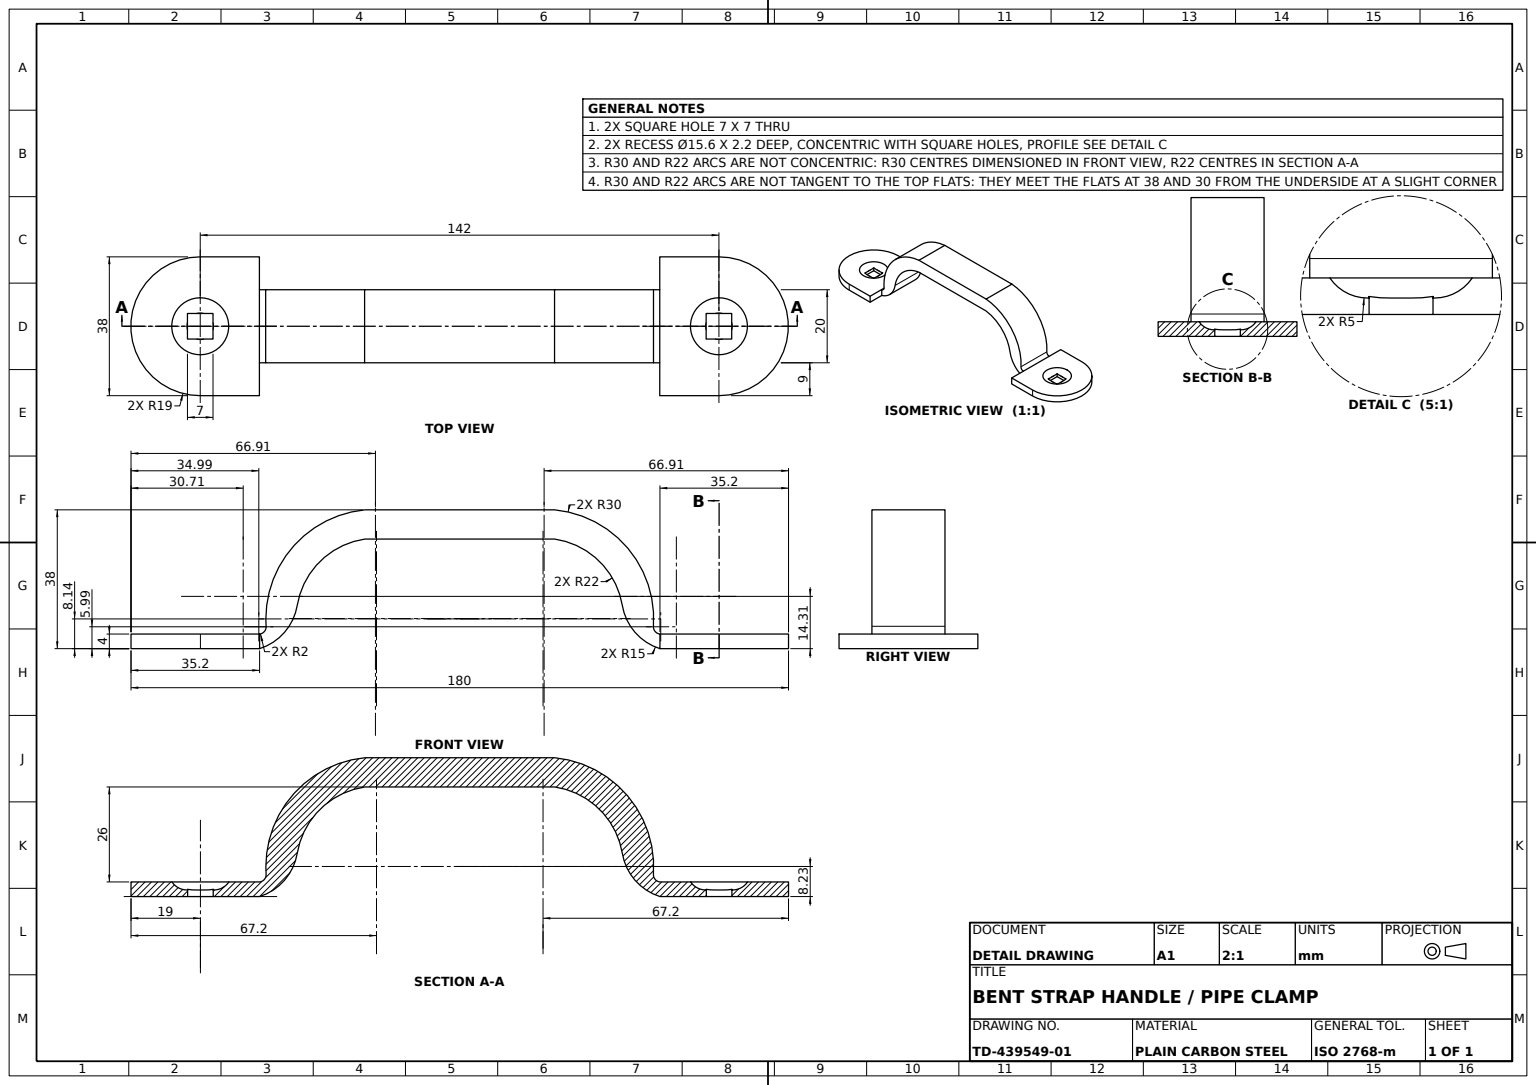
ISO-10303-21;
HEADER;
FILE_DESCRIPTION((''),'2;1');
FILE_NAME('','',(''),(''),'','','');
FILE_SCHEMA(('AUTOMOTIVE_DESIGN'));
ENDSEC;
DATA;
#1=APPLICATION_CONTEXT('');
#2=PRODUCT_CONTEXT('',#1,'mechanical');
#3=PRODUCT('','','',(#2));
#4=PRODUCT_DEFINITION_FORMATION('','',#3);
#5=PRODUCT_DEFINITION_CONTEXT('',#1,'design');
#6=PRODUCT_DEFINITION('','',#4,#5);
#7=PRODUCT_DEFINITION_SHAPE('','',#6);
#8=(LENGTH_UNIT()NAMED_UNIT(*)SI_UNIT(.MILLI.,.METRE.));
#9=(NAMED_UNIT(*)PLANE_ANGLE_UNIT()SI_UNIT($,.RADIAN.));
#10=(NAMED_UNIT(*)SI_UNIT($,.STERADIAN.)SOLID_ANGLE_UNIT());
#11=UNCERTAINTY_MEASURE_WITH_UNIT(LENGTH_MEASURE(1.E-05),#8,'distance_accuracy_value','');
#12=(GEOMETRIC_REPRESENTATION_CONTEXT(3)GLOBAL_UNCERTAINTY_ASSIGNED_CONTEXT((#11))GLOBAL_UNIT_ASSIGNED_CONTEXT((#8,#9,#10))REPRESENTATION_CONTEXT('',''));
#13=CARTESIAN_POINT('',(-16.2,4.,-19.));
#14=VERTEX_POINT('',#13);
#15=CARTESIAN_POINT('',(-16.2,4.,19.));
#16=VERTEX_POINT('',#15);
#17=CARTESIAN_POINT('',(-16.2,4.,0.));
#18=DIRECTION('',(0.,1.,0.));
#19=DIRECTION('',(0.,0.,1.));
#20=AXIS2_PLACEMENT_3D('',#17,#18,#19);
#21=CIRCLE('',#20,19.);
#22=EDGE_CURVE('',#14,#16,#21,.T.);
#23=ORIENTED_EDGE('',*,*,#22,.T.);
#24=CARTESIAN_POINT('',(0.,4.,19.));
#25=VERTEX_POINT('',#24);
#26=DIRECTION('',(1.,0.,0.));
#27=VECTOR('',#26,1000.);
#28=LINE('',#24,#27);
#29=EDGE_CURVE('',#16,#25,#28,.T.);
#30=ORIENTED_EDGE('',*,*,#29,.T.);
#31=CARTESIAN_POINT('',(0.,4.,10.));
#32=VERTEX_POINT('',#31);
#33=DIRECTION('',(0.,0.,-1.));
#34=VECTOR('',#33,1000.);
#35=LINE('',#24,#34);
#36=EDGE_CURVE('',#25,#32,#35,.T.);
#37=ORIENTED_EDGE('',*,*,#36,.T.);
#38=CARTESIAN_POINT('',(0.,4.,-10.));
#39=VERTEX_POINT('',#38);
#40=LINE('',#31,#34);
#41=EDGE_CURVE('',#32,#39,#40,.T.);
#42=ORIENTED_EDGE('',*,*,#41,.T.);
#43=CARTESIAN_POINT('',(0.,4.,-19.));
#44=VERTEX_POINT('',#43);
#45=EDGE_CURVE('',#39,#44,#35,.T.);
#46=ORIENTED_EDGE('',*,*,#45,.T.);
#47=DIRECTION('',(-1.,0.,0.));
#48=VECTOR('',#47,1000.);
#49=LINE('',#43,#48);
#50=EDGE_CURVE('',#44,#14,#49,.T.);
#51=ORIENTED_EDGE('',*,*,#50,.T.);
#52=EDGE_LOOP('',(#23,#30,#37,#42,#46,#51));
#53=FACE_OUTER_BOUND('',#52,.T.);
#54=CARTESIAN_POINT('',(-16.2,4.,7.8));
#55=VERTEX_POINT('',#54);
#56=CARTESIAN_POINT('',(-16.2,4.,-7.8));
#57=VERTEX_POINT('',#56);
#58=CIRCLE('',#20,7.8);
#59=EDGE_CURVE('',#55,#57,#58,.T.);
#60=ORIENTED_EDGE('',*,*,#59,.F.);
#61=EDGE_CURVE('',#57,#55,#58,.T.);
#62=ORIENTED_EDGE('',*,*,#61,.F.);
#63=EDGE_LOOP('',(#60,#62));
#64=FACE_BOUND('',#63,.T.);
#65=PLANE('',#20);
#66=ADVANCED_FACE('',(#53,#64),#65,.T.);
#67=CARTESIAN_POINT('',(107.814744,5.988438,-10.));
#68=VERTEX_POINT('',#67);
#69=CARTESIAN_POINT('',(107.819278,6.123019,-10.));
#70=VERTEX_POINT('',#69);
#71=CARTESIAN_POINT('',(109.814744,5.988438,-10.));
#72=AXIS2_PLACEMENT_3D('',#71,#33,#47);
#73=CIRCLE('',#72,2.);
#74=EDGE_CURVE('',#68,#70,#73,.T.);
#75=ORIENTED_EDGE('',*,*,#74,.T.);
#76=CARTESIAN_POINT('',(107.819278,6.123019,10.));
#77=VERTEX_POINT('',#76);
#78=LINE('',#76,#34);
#79=EDGE_CURVE('',#77,#70,#78,.T.);
#80=ORIENTED_EDGE('',*,*,#79,.F.);
#81=CARTESIAN_POINT('',(107.814744,5.988438,10.));
#82=VERTEX_POINT('',#81);
#83=CARTESIAN_POINT('',(109.814744,5.988438,10.));
#84=AXIS2_PLACEMENT_3D('',#83,#33,#47);
#85=CIRCLE('',#84,2.);
#86=EDGE_CURVE('',#82,#77,#85,.T.);
#87=ORIENTED_EDGE('',*,*,#86,.F.);
#88=LINE('',#81,#34);
#89=EDGE_CURVE('',#82,#68,#88,.T.);
#90=ORIENTED_EDGE('',*,*,#89,.T.);
#91=EDGE_LOOP('',(#75,#80,#87,#90));
#92=FACE_OUTER_BOUND('',#91,.T.);
#93=CYLINDRICAL_SURFACE('',#84,2.);
#94=ADVANCED_FACE('',(#92),#93,.F.);
#95=CARTESIAN_POINT('',(-12.7,1.8,1.061874));
#96=VERTEX_POINT('',#95);
#97=CARTESIAN_POINT('',(-12.7,1.8,-1.061874));
#98=VERTEX_POINT('',#97);
#99=CARTESIAN_POINT('',(-12.7,1.8,3.5));
#100=LINE('',#99,#34);
#101=EDGE_CURVE('',#96,#98,#100,.T.);
#102=ORIENTED_EDGE('',*,*,#101,.F.);
#103=CARTESIAN_POINT('',(-16.2,1.8,0.));
#104=AXIS2_PLACEMENT_3D('',#103,#18,#19);
#105=CIRCLE('',#104,3.657537);
#106=EDGE_CURVE('',#96,#98,#105,.T.);
#107=ORIENTED_EDGE('',*,*,#106,.T.);
#108=EDGE_LOOP('',(#102,#107));
#109=FACE_OUTER_BOUND('',#108,.T.);
#110=PLANE('',#104);
#111=ADVANCED_FACE('',(#109),#110,.T.);
#112=CARTESIAN_POINT('',(-19.7,0.,3.5));
#113=VERTEX_POINT('',#112);
#114=CARTESIAN_POINT('',(-12.7,0.,3.5));
#115=VERTEX_POINT('',#114);
#116=LINE('',#112,#27);
#117=EDGE_CURVE('',#113,#115,#116,.T.);
#118=ORIENTED_EDGE('',*,*,#117,.T.);
#119=CARTESIAN_POINT('',(-12.7,0.,-3.5));
#120=VERTEX_POINT('',#119);
#121=LINE('',#114,#34);
#122=EDGE_CURVE('',#115,#120,#121,.T.);
#123=ORIENTED_EDGE('',*,*,#122,.T.);
#124=CARTESIAN_POINT('',(-19.7,0.,-3.5));
#125=VERTEX_POINT('',#124);
#126=LINE('',#124,#48);
#127=EDGE_CURVE('',#120,#125,#126,.T.);
#128=ORIENTED_EDGE('',*,*,#127,.T.);
#129=VECTOR('',#19,1000.);
#130=LINE('',#112,#129);
#131=EDGE_CURVE('',#125,#113,#130,.T.);
#132=ORIENTED_EDGE('',*,*,#131,.T.);
#133=EDGE_LOOP('',(#118,#123,#128,#132));
#134=FACE_BOUND('',#133,.T.);
#135=CARTESIAN_POINT('',(0.,0.,-10.));
#136=VERTEX_POINT('',#135);
#137=CARTESIAN_POINT('',(0.,0.,-19.));
#138=VERTEX_POINT('',#137);
#139=CARTESIAN_POINT('',(0.,0.,19.));
#140=LINE('',#139,#34);
#141=EDGE_CURVE('',#136,#138,#140,.T.);
#142=ORIENTED_EDGE('',*,*,#141,.F.);
#143=CARTESIAN_POINT('',(0.,0.,10.));
#144=VERTEX_POINT('',#143);
#145=LINE('',#143,#34);
#146=EDGE_CURVE('',#144,#136,#145,.T.);
#147=ORIENTED_EDGE('',*,*,#146,.F.);
#148=VERTEX_POINT('',#139);
#149=EDGE_CURVE('',#148,#144,#140,.T.);
#150=ORIENTED_EDGE('',*,*,#149,.F.);
#151=CARTESIAN_POINT('',(-16.2,0.,19.));
#152=VERTEX_POINT('',#151);
#153=LINE('',#139,#27);
#154=EDGE_CURVE('',#152,#148,#153,.T.);
#155=ORIENTED_EDGE('',*,*,#154,.F.);
#156=CARTESIAN_POINT('',(-16.2,0.,-19.));
#157=VERTEX_POINT('',#156);
#158=CARTESIAN_POINT('',(-16.2,0.,0.));
#159=AXIS2_PLACEMENT_3D('',#158,#18,#19);
#160=CIRCLE('',#159,19.);
#161=EDGE_CURVE('',#157,#152,#160,.T.);
#162=ORIENTED_EDGE('',*,*,#161,.F.);
#163=LINE('',#137,#48);
#164=EDGE_CURVE('',#138,#157,#163,.T.);
#165=ORIENTED_EDGE('',*,*,#164,.F.);
#166=EDGE_LOOP('',(#142,#147,#150,#155,#162,#165));
#167=FACE_OUTER_BOUND('',#166,.T.);
#168=PLANE('',#159);
#169=ADVANCED_FACE('',(#134,#167),#168,.F.);
#170=CARTESIAN_POINT('',(109.6,0.,-19.));
#171=VERTEX_POINT('',#170);
#172=CARTESIAN_POINT('',(109.6,0.,-10.));
#173=VERTEX_POINT('',#172);
#174=CARTESIAN_POINT('',(109.6,0.,19.));
#175=LINE('',#174,#129);
#176=EDGE_CURVE('',#171,#173,#175,.T.);
#177=ORIENTED_EDGE('',*,*,#176,.T.);
#178=CARTESIAN_POINT('',(109.6,4.,-10.));
#179=VERTEX_POINT('',#178);
#180=VECTOR('',#18,1000.);
#181=LINE('',#172,#180);
#182=EDGE_CURVE('',#173,#179,#181,.T.);
#183=ORIENTED_EDGE('',*,*,#182,.T.);
#184=CARTESIAN_POINT('',(109.6,4.,-19.));
#185=VERTEX_POINT('',#184);
#186=CARTESIAN_POINT('',(109.6,4.,19.));
#187=LINE('',#186,#129);
#188=EDGE_CURVE('',#185,#179,#187,.T.);
#189=ORIENTED_EDGE('',*,*,#188,.F.);
#190=DIRECTION('',(0.,-1.,0.));
#191=VECTOR('',#190,1000.);
#192=LINE('',#184,#191);
#193=EDGE_CURVE('',#185,#171,#192,.T.);
#194=ORIENTED_EDGE('',*,*,#193,.T.);
#195=EDGE_LOOP('',(#177,#183,#189,#194));
#196=FACE_OUTER_BOUND('',#195,.T.);
#197=AXIS2_PLACEMENT_3D('',#186,#26,#33);
#198=PLANE('',#197);
#199=ADVANCED_FACE('',(#196),#198,.F.);
#200=CARTESIAN_POINT('',(122.3,1.8,-1.061874));
#201=VERTEX_POINT('',#200);
#202=CARTESIAN_POINT('',(122.3,1.8,1.061874));
#203=VERTEX_POINT('',#202);
#204=CARTESIAN_POINT('',(125.8,1.8,0.));
#205=AXIS2_PLACEMENT_3D('',#204,#18,#33);
#206=CIRCLE('',#205,3.657537);
#207=EDGE_CURVE('',#201,#203,#206,.T.);
#208=ORIENTED_EDGE('',*,*,#207,.T.);
#209=CARTESIAN_POINT('',(122.3,1.8,3.5));
#210=LINE('',#209,#129);
#211=EDGE_CURVE('',#201,#203,#210,.T.);
#212=ORIENTED_EDGE('',*,*,#211,.F.);
#213=EDGE_LOOP('',(#208,#212));
#214=FACE_OUTER_BOUND('',#213,.T.);
#215=AXIS2_PLACEMENT_3D('',#204,#190,#33);
#216=PLANE('',#215);
#217=ADVANCED_FACE('',(#214),#216,.F.);
#218=CARTESIAN_POINT('',(28.8,38.,10.));
#219=VERTEX_POINT('',#218);
#220=CARTESIAN_POINT('',(28.8,38.,-10.));
#221=VERTEX_POINT('',#220);
#222=LINE('',#218,#34);
#223=EDGE_CURVE('',#219,#221,#222,.T.);
#224=ORIENTED_EDGE('',*,*,#223,.T.);
#225=CARTESIAN_POINT('',(1.712725,8.141734,-10.));
#226=VERTEX_POINT('',#225);
#227=CARTESIAN_POINT('',(31.712725,8.141734,-10.));
#228=AXIS2_PLACEMENT_3D('',#227,#19,#47);
#229=CIRCLE('',#228,30.);
#230=EDGE_CURVE('',#221,#226,#229,.T.);
#231=ORIENTED_EDGE('',*,*,#230,.T.);
#232=CARTESIAN_POINT('',(1.712725,8.141734,10.));
#233=VERTEX_POINT('',#232);
#234=LINE('',#232,#34);
#235=EDGE_CURVE('',#233,#226,#234,.T.);
#236=ORIENTED_EDGE('',*,*,#235,.F.);
#237=CARTESIAN_POINT('',(31.712725,8.141734,10.));
#238=AXIS2_PLACEMENT_3D('',#237,#19,#47);
#239=CIRCLE('',#238,30.);
#240=EDGE_CURVE('',#219,#233,#239,.T.);
#241=ORIENTED_EDGE('',*,*,#240,.F.);
#242=EDGE_LOOP('',(#224,#231,#236,#241));
#243=FACE_OUTER_BOUND('',#242,.T.);
#244=AXIS2_PLACEMENT_3D('',#237,#33,#47);
#245=CYLINDRICAL_SURFACE('',#244,30.);
#246=ADVANCED_FACE('',(#243),#245,.T.);
#247=CARTESIAN_POINT('',(124.738126,1.8,3.5));
#248=VERTEX_POINT('',#247);
#249=CARTESIAN_POINT('',(125.8,1.8,3.657537));
#250=VERTEX_POINT('',#249);
#251=EDGE_CURVE('',#248,#250,#206,.T.);
#252=ORIENTED_EDGE('',*,*,#251,.T.);
#253=CARTESIAN_POINT('',(126.861874,1.8,3.5));
#254=VERTEX_POINT('',#253);
#255=EDGE_CURVE('',#250,#254,#206,.T.);
#256=ORIENTED_EDGE('',*,*,#255,.T.);
#257=LINE('',#209,#27);
#258=EDGE_CURVE('',#248,#254,#257,.T.);
#259=ORIENTED_EDGE('',*,*,#258,.F.);
#260=EDGE_LOOP('',(#252,#256,#259));
#261=FACE_OUTER_BOUND('',#260,.T.);
#262=ADVANCED_FACE('',(#261),#216,.F.);
#263=CARTESIAN_POINT('',(125.8,4.,7.8));
#264=VERTEX_POINT('',#263);
#265=CARTESIAN_POINT('',(125.8,6.8,3.657537));
#266=AXIS2_PLACEMENT_3D('',#265,#47,#19);
#267=CIRCLE('',#266,5.);
#268=EDGE_CURVE('',#250,#264,#267,.T.);
#269=ORIENTED_EDGE('',*,*,#268,.F.);
#270=ORIENTED_EDGE('',*,*,#251,.F.);
#271=CARTESIAN_POINT('',(122.3,1.969866,3.5));
#272=VERTEX_POINT('',#271);
#273=CARTESIAN_POINT('',(123.10603,1.817387,3.5));
#274=CARTESIAN_POINT('',(123.921472,1.8,3.5));
#275=B_SPLINE_CURVE_WITH_KNOTS('',3,(#271,#273,#274,#247),.UNSPECIFIED.,.F.,.F.,(4,4),(0.,0.002444036),.UNSPECIFIED.);
#276=EDGE_CURVE('',#272,#248,#275,.T.);
#277=ORIENTED_EDGE('',*,*,#276,.F.);
#278=CARTESIAN_POINT('',(122.3,1.8,1.878528));
#279=CARTESIAN_POINT('',(122.3,1.817387,2.69397));
#280=B_SPLINE_CURVE_WITH_KNOTS('',3,(#202,#278,#279,#271),.UNSPECIFIED.,.F.,.F.,(4,4),(0.,0.002444036),.UNSPECIFIED.);
#281=EDGE_CURVE('',#203,#272,#280,.T.);
#282=ORIENTED_EDGE('',*,*,#281,.F.);
#283=ORIENTED_EDGE('',*,*,#207,.F.);
#284=CARTESIAN_POINT('',(122.3,1.969866,-3.5));
#285=VERTEX_POINT('',#284);
#286=CARTESIAN_POINT('',(122.3,1.817387,-2.69397));
#287=CARTESIAN_POINT('',(122.3,1.8,-1.878528));
#288=B_SPLINE_CURVE_WITH_KNOTS('',3,(#284,#286,#287,#200),.UNSPECIFIED.,.F.,.F.,(4,4),(0.,0.002444036),.UNSPECIFIED.);
#289=EDGE_CURVE('',#285,#201,#288,.T.);
#290=ORIENTED_EDGE('',*,*,#289,.F.);
#291=CARTESIAN_POINT('',(124.738126,1.8,-3.5));
#292=VERTEX_POINT('',#291);
#293=CARTESIAN_POINT('',(123.921472,1.8,-3.5));
#294=CARTESIAN_POINT('',(123.10603,1.817387,-3.5));
#295=B_SPLINE_CURVE_WITH_KNOTS('',3,(#291,#293,#294,#284),.UNSPECIFIED.,.F.,.F.,(4,4),(0.,0.002444036),.UNSPECIFIED.);
#296=EDGE_CURVE('',#292,#285,#295,.T.);
#297=ORIENTED_EDGE('',*,*,#296,.F.);
#298=CARTESIAN_POINT('',(125.8,1.8,-3.657537));
#299=VERTEX_POINT('',#298);
#300=EDGE_CURVE('',#299,#292,#206,.T.);
#301=ORIENTED_EDGE('',*,*,#300,.F.);
#302=CARTESIAN_POINT('',(125.8,4.,-7.8));
#303=VERTEX_POINT('',#302);
#304=CARTESIAN_POINT('',(125.8,6.8,-3.657537));
#305=AXIS2_PLACEMENT_3D('',#304,#26,#33);
#306=CIRCLE('',#305,5.);
#307=EDGE_CURVE('',#299,#303,#306,.T.);
#308=ORIENTED_EDGE('',*,*,#307,.T.);
#309=CARTESIAN_POINT('',(125.8,4.,0.));
#310=AXIS2_PLACEMENT_3D('',#309,#18,#33);
#311=CIRCLE('',#310,7.8);
#312=EDGE_CURVE('',#303,#264,#311,.T.);
#313=ORIENTED_EDGE('',*,*,#312,.T.);
#314=EDGE_LOOP('',(#269,#270,#277,#282,#283,#290,#297,#301,#308,#313));
#315=FACE_OUTER_BOUND('',#314,.T.);
#316=CARTESIAN_POINT('',(125.8,6.8,0.));
#317=AXIS2_PLACEMENT_3D('',#316,#18,#19);
#318=TOROIDAL_SURFACE('',#317,3.657537,5.);
#319=ADVANCED_FACE('',(#315),#318,.F.);
#320=CARTESIAN_POINT('',(80.8,38.,10.));
#321=VERTEX_POINT('',#320);
#322=LINE('',#218,#48);
#323=EDGE_CURVE('',#321,#219,#322,.T.);
#324=ORIENTED_EDGE('',*,*,#323,.F.);
#325=CARTESIAN_POINT('',(80.8,38.,-10.));
#326=VERTEX_POINT('',#325);
#327=LINE('',#320,#34);
#328=EDGE_CURVE('',#321,#326,#327,.T.);
#329=ORIENTED_EDGE('',*,*,#328,.T.);
#330=LINE('',#220,#48);
#331=EDGE_CURVE('',#326,#221,#330,.T.);
#332=ORIENTED_EDGE('',*,*,#331,.T.);
#333=ORIENTED_EDGE('',*,*,#223,.F.);
#334=EDGE_LOOP('',(#324,#329,#332,#333));
#335=FACE_OUTER_BOUND('',#334,.T.);
#336=AXIS2_PLACEMENT_3D('',#218,#190,#26);
#337=PLANE('',#336);
#338=ADVANCED_FACE('',(#335),#337,.F.);
#339=EDGE_CURVE('',#264,#303,#311,.T.);
#340=ORIENTED_EDGE('',*,*,#339,.F.);
#341=ORIENTED_EDGE('',*,*,#312,.F.);
#342=EDGE_LOOP('',(#340,#341));
#343=FACE_BOUND('',#342,.T.);
#344=ORIENTED_EDGE('',*,*,#188,.T.);
#345=CARTESIAN_POINT('',(109.6,4.,10.));
#346=VERTEX_POINT('',#345);
#347=LINE('',#345,#34);
#348=EDGE_CURVE('',#346,#179,#347,.T.);
#349=ORIENTED_EDGE('',*,*,#348,.F.);
#350=VERTEX_POINT('',#186);
#351=EDGE_CURVE('',#346,#350,#187,.T.);
#352=ORIENTED_EDGE('',*,*,#351,.T.);
#353=CARTESIAN_POINT('',(125.8,4.,19.));
#354=VERTEX_POINT('',#353);
#355=LINE('',#186,#27);
#356=EDGE_CURVE('',#350,#354,#355,.T.);
#357=ORIENTED_EDGE('',*,*,#356,.T.);
#358=CARTESIAN_POINT('',(125.8,4.,-19.));
#359=VERTEX_POINT('',#358);
#360=CIRCLE('',#310,19.);
#361=EDGE_CURVE('',#354,#359,#360,.T.);
#362=ORIENTED_EDGE('',*,*,#361,.T.);
#363=LINE('',#184,#48);
#364=EDGE_CURVE('',#359,#185,#363,.T.);
#365=ORIENTED_EDGE('',*,*,#364,.T.);
#366=EDGE_LOOP('',(#344,#349,#352,#357,#362,#365));
#367=FACE_OUTER_BOUND('',#366,.T.);
#368=AXIS2_PLACEMENT_3D('',#309,#190,#33);
#369=PLANE('',#368);
#370=ADVANCED_FACE('',(#343,#367),#369,.F.);
#371=ORIENTED_EDGE('',*,*,#106,.F.);
#372=CARTESIAN_POINT('',(-12.7,1.969866,3.5));
#373=VERTEX_POINT('',#372);
#374=CARTESIAN_POINT('',(-12.7,1.817387,2.69397));
#375=CARTESIAN_POINT('',(-12.7,1.8,1.878528));
#376=B_SPLINE_CURVE_WITH_KNOTS('',3,(#372,#374,#375,#95),.UNSPECIFIED.,.F.,.F.,(4,4),(0.,0.002444036),.UNSPECIFIED.);
#377=EDGE_CURVE('',#373,#96,#376,.T.);
#378=ORIENTED_EDGE('',*,*,#377,.F.);
#379=CARTESIAN_POINT('',(-15.138126,1.8,3.5));
#380=VERTEX_POINT('',#379);
#381=CARTESIAN_POINT('',(-14.321472,1.8,3.5));
#382=CARTESIAN_POINT('',(-13.50603,1.817387,3.5));
#383=B_SPLINE_CURVE_WITH_KNOTS('',3,(#379,#381,#382,#372),.UNSPECIFIED.,.F.,.F.,(4,4),(0.,0.002444036),.UNSPECIFIED.);
#384=EDGE_CURVE('',#380,#373,#383,.T.);
#385=ORIENTED_EDGE('',*,*,#384,.F.);
#386=CARTESIAN_POINT('',(-16.2,1.8,3.657537));
#387=VERTEX_POINT('',#386);
#388=EDGE_CURVE('',#387,#380,#105,.T.);
#389=ORIENTED_EDGE('',*,*,#388,.F.);
#390=CARTESIAN_POINT('',(-16.2,6.8,3.657537));
#391=AXIS2_PLACEMENT_3D('',#390,#26,#33);
#392=CIRCLE('',#391,5.);
#393=EDGE_CURVE('',#55,#387,#392,.T.);
#394=ORIENTED_EDGE('',*,*,#393,.F.);
#395=ORIENTED_EDGE('',*,*,#59,.T.);
#396=CARTESIAN_POINT('',(-16.2,1.8,-3.657537));
#397=VERTEX_POINT('',#396);
#398=CARTESIAN_POINT('',(-16.2,6.8,-3.657537));
#399=AXIS2_PLACEMENT_3D('',#398,#47,#19);
#400=CIRCLE('',#399,5.);
#401=EDGE_CURVE('',#57,#397,#400,.T.);
#402=ORIENTED_EDGE('',*,*,#401,.T.);
#403=CARTESIAN_POINT('',(-15.138126,1.8,-3.5));
#404=VERTEX_POINT('',#403);
#405=EDGE_CURVE('',#404,#397,#105,.T.);
#406=ORIENTED_EDGE('',*,*,#405,.F.);
#407=CARTESIAN_POINT('',(-12.7,1.969866,-3.5));
#408=VERTEX_POINT('',#407);
#409=CARTESIAN_POINT('',(-13.50603,1.817387,-3.5));
#410=CARTESIAN_POINT('',(-14.321472,1.8,-3.5));
#411=B_SPLINE_CURVE_WITH_KNOTS('',3,(#407,#409,#410,#403),.UNSPECIFIED.,.F.,.F.,(4,4),(0.,0.002444036),.UNSPECIFIED.);
#412=EDGE_CURVE('',#408,#404,#411,.T.);
#413=ORIENTED_EDGE('',*,*,#412,.F.);
#414=CARTESIAN_POINT('',(-12.7,1.8,-1.878528));
#415=CARTESIAN_POINT('',(-12.7,1.817387,-2.69397));
#416=B_SPLINE_CURVE_WITH_KNOTS('',3,(#97,#414,#415,#407),.UNSPECIFIED.,.F.,.F.,(4,4),(0.,0.002444036),.UNSPECIFIED.);
#417=EDGE_CURVE('',#98,#408,#416,.T.);
#418=ORIENTED_EDGE('',*,*,#417,.F.);
#419=EDGE_LOOP('',(#371,#378,#385,#389,#394,#395,#402,#406,#413,#418));
#420=FACE_OUTER_BOUND('',#419,.T.);
#421=CARTESIAN_POINT('',(-16.2,6.8,0.));
#422=AXIS2_PLACEMENT_3D('',#421,#190,#33);
#423=TOROIDAL_SURFACE('',#422,3.657537,5.);
#424=ADVANCED_FACE('',(#420),#423,.F.);
#425=ORIENTED_EDGE('',*,*,#348,.T.);
#426=EDGE_CURVE('',#179,#68,#73,.T.);
#427=ORIENTED_EDGE('',*,*,#426,.T.);
#428=ORIENTED_EDGE('',*,*,#89,.F.);
#429=EDGE_CURVE('',#346,#82,#85,.T.);
#430=ORIENTED_EDGE('',*,*,#429,.F.);
#431=EDGE_LOOP('',(#425,#427,#428,#430));
#432=FACE_OUTER_BOUND('',#431,.T.);
#433=ADVANCED_FACE('',(#432),#93,.F.);
#434=CARTESIAN_POINT('',(99.296405,11.847852,-10.));
#435=VERTEX_POINT('',#434);
#436=CARTESIAN_POINT('',(114.092724,14.311374,-10.));
#437=AXIS2_PLACEMENT_3D('',#436,#19,#47);
#438=CIRCLE('',#437,15.);
#439=EDGE_CURVE('',#435,#173,#438,.T.);
#440=ORIENTED_EDGE('',*,*,#439,.T.);
#441=CARTESIAN_POINT('',(109.6,0.,10.));
#442=VERTEX_POINT('',#441);
#443=LINE('',#441,#34);
#444=EDGE_CURVE('',#442,#173,#443,.T.);
#445=ORIENTED_EDGE('',*,*,#444,.F.);
#446=CARTESIAN_POINT('',(99.296405,11.847852,10.));
#447=VERTEX_POINT('',#446);
#448=CARTESIAN_POINT('',(114.092724,14.311374,10.));
#449=AXIS2_PLACEMENT_3D('',#448,#19,#47);
#450=CIRCLE('',#449,15.);
#451=EDGE_CURVE('',#447,#442,#450,.T.);
#452=ORIENTED_EDGE('',*,*,#451,.F.);
#453=LINE('',#446,#34);
#454=EDGE_CURVE('',#447,#435,#453,.T.);
#455=ORIENTED_EDGE('',*,*,#454,.T.);
#456=EDGE_LOOP('',(#440,#445,#452,#455));
#457=FACE_OUTER_BOUND('',#456,.T.);
#458=AXIS2_PLACEMENT_3D('',#448,#33,#47);
#459=CYLINDRICAL_SURFACE('',#458,15.);
#460=ADVANCED_FACE('',(#457),#459,.T.);
#461=CARTESIAN_POINT('',(80.8,30.,10.));
#462=VERTEX_POINT('',#461);
#463=CARTESIAN_POINT('',(77.595137,8.234687,10.));
#464=AXIS2_PLACEMENT_3D('',#463,#33,#26);
#465=CIRCLE('',#464,22.);
#466=EDGE_CURVE('',#462,#447,#465,.T.);
#467=ORIENTED_EDGE('',*,*,#466,.F.);
#468=CARTESIAN_POINT('',(80.8,30.,-10.));
#469=VERTEX_POINT('',#468);
#470=LINE('',#461,#34);
#471=EDGE_CURVE('',#462,#469,#470,.T.);
#472=ORIENTED_EDGE('',*,*,#471,.T.);
#473=CARTESIAN_POINT('',(77.595137,8.234687,-10.));
#474=AXIS2_PLACEMENT_3D('',#473,#33,#26);
#475=CIRCLE('',#474,22.);
#476=EDGE_CURVE('',#469,#435,#475,.T.);
#477=ORIENTED_EDGE('',*,*,#476,.T.);
#478=ORIENTED_EDGE('',*,*,#454,.F.);
#479=EDGE_LOOP('',(#467,#472,#477,#478));
#480=FACE_OUTER_BOUND('',#479,.T.);
#481=AXIS2_PLACEMENT_3D('',#463,#33,#47);
#482=CYLINDRICAL_SURFACE('',#481,22.);
#483=ADVANCED_FACE('',(#480),#482,.F.);
#484=ORIENTED_EDGE('',*,*,#193,.F.);
#485=ORIENTED_EDGE('',*,*,#364,.F.);
#486=CARTESIAN_POINT('',(125.8,0.,-19.));
#487=VERTEX_POINT('',#486);
#488=LINE('',#358,#191);
#489=EDGE_CURVE('',#359,#487,#488,.T.);
#490=ORIENTED_EDGE('',*,*,#489,.T.);
#491=LINE('',#170,#48);
#492=EDGE_CURVE('',#487,#171,#491,.T.);
#493=ORIENTED_EDGE('',*,*,#492,.T.);
#494=EDGE_LOOP('',(#484,#485,#490,#493));
#495=FACE_OUTER_BOUND('',#494,.T.);
#496=AXIS2_PLACEMENT_3D('',#184,#19,#26);
#497=PLANE('',#496);
#498=ADVANCED_FACE('',(#495),#497,.F.);
#499=CARTESIAN_POINT('',(-19.7,1.8,-1.061874));
#500=VERTEX_POINT('',#499);
#501=CARTESIAN_POINT('',(-19.7,1.8,1.061874));
#502=VERTEX_POINT('',#501);
#503=CARTESIAN_POINT('',(-19.7,1.8,3.5));
#504=LINE('',#503,#129);
#505=EDGE_CURVE('',#500,#502,#504,.T.);
#506=ORIENTED_EDGE('',*,*,#505,.F.);
#507=EDGE_CURVE('',#500,#502,#105,.T.);
#508=ORIENTED_EDGE('',*,*,#507,.T.);
#509=EDGE_LOOP('',(#506,#508));
#510=FACE_OUTER_BOUND('',#509,.T.);
#511=ADVANCED_FACE('',(#510),#110,.T.);
#512=CARTESIAN_POINT('',(10.303595,11.847852,10.));
#513=VERTEX_POINT('',#512);
#514=CARTESIAN_POINT('',(-4.492724,14.311374,10.));
#515=AXIS2_PLACEMENT_3D('',#514,#19,#26);
#516=CIRCLE('',#515,15.);
#517=EDGE_CURVE('',#144,#513,#516,.T.);
#518=ORIENTED_EDGE('',*,*,#517,.F.);
#519=ORIENTED_EDGE('',*,*,#146,.T.);
#520=CARTESIAN_POINT('',(10.303595,11.847852,-10.));
#521=VERTEX_POINT('',#520);
#522=CARTESIAN_POINT('',(-4.492724,14.311374,-10.));
#523=AXIS2_PLACEMENT_3D('',#522,#19,#26);
#524=CIRCLE('',#523,15.);
#525=EDGE_CURVE('',#136,#521,#524,.T.);
#526=ORIENTED_EDGE('',*,*,#525,.T.);
#527=LINE('',#512,#34);
#528=EDGE_CURVE('',#513,#521,#527,.T.);
#529=ORIENTED_EDGE('',*,*,#528,.F.);
#530=EDGE_LOOP('',(#518,#519,#526,#529));
#531=FACE_OUTER_BOUND('',#530,.T.);
#532=AXIS2_PLACEMENT_3D('',#514,#33,#47);
#533=CYLINDRICAL_SURFACE('',#532,15.);
#534=ADVANCED_FACE('',(#531),#533,.T.);
#535=ORIENTED_EDGE('',*,*,#356,.F.);
#536=VERTEX_POINT('',#174);
#537=LINE('',#186,#191);
#538=EDGE_CURVE('',#350,#536,#537,.T.);
#539=ORIENTED_EDGE('',*,*,#538,.T.);
#540=CARTESIAN_POINT('',(125.8,0.,19.));
#541=VERTEX_POINT('',#540);
#542=LINE('',#174,#27);
#543=EDGE_CURVE('',#536,#541,#542,.T.);
#544=ORIENTED_EDGE('',*,*,#543,.T.);
#545=LINE('',#353,#191);
#546=EDGE_CURVE('',#354,#541,#545,.T.);
#547=ORIENTED_EDGE('',*,*,#546,.F.);
#548=EDGE_LOOP('',(#535,#539,#544,#547));
#549=FACE_OUTER_BOUND('',#548,.T.);
#550=AXIS2_PLACEMENT_3D('',#186,#33,#47);
#551=PLANE('',#550);
#552=ADVANCED_FACE('',(#549),#551,.F.);
#553=CARTESIAN_POINT('',(1.780722,6.123019,10.));
#554=VERTEX_POINT('',#553);
#555=EDGE_CURVE('',#233,#554,#239,.T.);
#556=ORIENTED_EDGE('',*,*,#555,.F.);
#557=ORIENTED_EDGE('',*,*,#235,.T.);
#558=CARTESIAN_POINT('',(1.780722,6.123019,-10.));
#559=VERTEX_POINT('',#558);
#560=EDGE_CURVE('',#226,#559,#229,.T.);
#561=ORIENTED_EDGE('',*,*,#560,.T.);
#562=LINE('',#553,#34);
#563=EDGE_CURVE('',#554,#559,#562,.T.);
#564=ORIENTED_EDGE('',*,*,#563,.F.);
#565=EDGE_LOOP('',(#556,#557,#561,#564));
#566=FACE_OUTER_BOUND('',#565,.T.);
#567=ADVANCED_FACE('',(#566),#245,.T.);
#568=LINE('',#31,#191);
#569=EDGE_CURVE('',#32,#144,#568,.T.);
#570=ORIENTED_EDGE('',*,*,#569,.T.);
#571=ORIENTED_EDGE('',*,*,#517,.T.);
#572=CARTESIAN_POINT('',(28.8,30.,10.));
#573=VERTEX_POINT('',#572);
#574=CARTESIAN_POINT('',(32.004863,8.234687,10.));
#575=AXIS2_PLACEMENT_3D('',#574,#33,#47);
#576=CIRCLE('',#575,22.);
#577=EDGE_CURVE('',#513,#573,#576,.T.);
#578=ORIENTED_EDGE('',*,*,#577,.T.);
#579=LINE('',#572,#27);
#580=EDGE_CURVE('',#573,#462,#579,.T.);
#581=ORIENTED_EDGE('',*,*,#580,.T.);
#582=ORIENTED_EDGE('',*,*,#466,.T.);
#583=ORIENTED_EDGE('',*,*,#451,.T.);
#584=LINE('',#441,#180);
#585=EDGE_CURVE('',#442,#346,#584,.T.);
#586=ORIENTED_EDGE('',*,*,#585,.T.);
#587=ORIENTED_EDGE('',*,*,#429,.T.);
#588=ORIENTED_EDGE('',*,*,#86,.T.);
#589=CARTESIAN_POINT('',(77.887275,8.141734,10.));
#590=AXIS2_PLACEMENT_3D('',#589,#19,#26);
#591=CIRCLE('',#590,30.);
#592=EDGE_CURVE('',#77,#321,#591,.T.);
#593=ORIENTED_EDGE('',*,*,#592,.T.);
#594=ORIENTED_EDGE('',*,*,#323,.T.);
#595=ORIENTED_EDGE('',*,*,#240,.T.);
#596=ORIENTED_EDGE('',*,*,#555,.T.);
#597=CARTESIAN_POINT('',(-0.214744,5.988438,10.));
#598=AXIS2_PLACEMENT_3D('',#597,#33,#26);
#599=CIRCLE('',#598,2.);
#600=EDGE_CURVE('',#554,#32,#599,.T.);
#601=ORIENTED_EDGE('',*,*,#600,.T.);
#602=EDGE_LOOP('',(#570,#571,#578,#581,#582,#583,#586,#587,#588,#593,#594,#595,#596,#601));
#603=FACE_OUTER_BOUND('',#602,.T.);
#604=PLANE('',#515);
#605=ADVANCED_FACE('',(#603),#604,.T.);
#606=CARTESIAN_POINT('',(-0.214744,5.988438,-10.));
#607=AXIS2_PLACEMENT_3D('',#606,#33,#26);
#608=CIRCLE('',#607,2.);
#609=EDGE_CURVE('',#559,#39,#608,.T.);
#610=ORIENTED_EDGE('',*,*,#609,.T.);
#611=ORIENTED_EDGE('',*,*,#41,.F.);
#612=ORIENTED_EDGE('',*,*,#600,.F.);
#613=ORIENTED_EDGE('',*,*,#563,.T.);
#614=EDGE_LOOP('',(#610,#611,#612,#613));
#615=FACE_OUTER_BOUND('',#614,.T.);
#616=AXIS2_PLACEMENT_3D('',#597,#33,#47);
#617=CYLINDRICAL_SURFACE('',#616,2.);
#618=ADVANCED_FACE('',(#615),#617,.F.);
#619=CARTESIAN_POINT('',(129.3,0.,-3.5));
#620=VERTEX_POINT('',#619);
#621=CARTESIAN_POINT('',(129.3,1.969866,-3.5));
#622=VERTEX_POINT('',#621);
#623=LINE('',#619,#180);
#624=EDGE_CURVE('',#620,#622,#623,.T.);
#625=ORIENTED_EDGE('',*,*,#624,.F.);
#626=CARTESIAN_POINT('',(129.3,0.,3.5));
#627=VERTEX_POINT('',#626);
#628=LINE('',#626,#34);
#629=EDGE_CURVE('',#627,#620,#628,.T.);
#630=ORIENTED_EDGE('',*,*,#629,.F.);
#631=CARTESIAN_POINT('',(129.3,1.969866,3.5));
#632=VERTEX_POINT('',#631);
#633=LINE('',#626,#180);
#634=EDGE_CURVE('',#627,#632,#633,.T.);
#635=ORIENTED_EDGE('',*,*,#634,.T.);
#636=CARTESIAN_POINT('',(129.3,1.8,1.061874));
#637=VERTEX_POINT('',#636);
#638=CARTESIAN_POINT('',(129.3,1.817387,2.69397));
#639=CARTESIAN_POINT('',(129.3,1.8,1.878528));
#640=B_SPLINE_CURVE_WITH_KNOTS('',3,(#631,#638,#639,#636),.UNSPECIFIED.,.F.,.F.,(4,4),(0.,0.002444036),.UNSPECIFIED.);
#641=EDGE_CURVE('',#632,#637,#640,.T.);
#642=ORIENTED_EDGE('',*,*,#641,.T.);
#643=CARTESIAN_POINT('',(129.3,1.8,-1.061874));
#644=VERTEX_POINT('',#643);
#645=CARTESIAN_POINT('',(129.3,1.8,3.5));
#646=LINE('',#645,#34);
#647=EDGE_CURVE('',#637,#644,#646,.T.);
#648=ORIENTED_EDGE('',*,*,#647,.T.);
#649=CARTESIAN_POINT('',(129.3,1.8,-1.878528));
#650=CARTESIAN_POINT('',(129.3,1.817387,-2.69397));
#651=B_SPLINE_CURVE_WITH_KNOTS('',3,(#643,#649,#650,#621),.UNSPECIFIED.,.F.,.F.,(4,4),(0.,0.002444036),.UNSPECIFIED.);
#652=EDGE_CURVE('',#644,#622,#651,.T.);
#653=ORIENTED_EDGE('',*,*,#652,.T.);
#654=EDGE_LOOP('',(#625,#630,#635,#642,#648,#653));
#655=FACE_OUTER_BOUND('',#654,.T.);
#656=AXIS2_PLACEMENT_3D('',#626,#26,#33);
#657=PLANE('',#656);
#658=ADVANCED_FACE('',(#655),#657,.F.);
#659=LINE('',#114,#180);
#660=EDGE_CURVE('',#115,#373,#659,.T.);
#661=ORIENTED_EDGE('',*,*,#660,.F.);
#662=ORIENTED_EDGE('',*,*,#117,.F.);
#663=CARTESIAN_POINT('',(-19.7,1.969866,3.5));
#664=VERTEX_POINT('',#663);
#665=LINE('',#112,#180);
#666=EDGE_CURVE('',#113,#664,#665,.T.);
#667=ORIENTED_EDGE('',*,*,#666,.T.);
#668=CARTESIAN_POINT('',(-17.261874,1.8,3.5));
#669=VERTEX_POINT('',#668);
#670=CARTESIAN_POINT('',(-18.89397,1.817387,3.5));
#671=CARTESIAN_POINT('',(-18.078528,1.8,3.5));
#672=B_SPLINE_CURVE_WITH_KNOTS('',3,(#663,#670,#671,#668),.UNSPECIFIED.,.F.,.F.,(4,4),(0.,0.002444036),.UNSPECIFIED.);
#673=EDGE_CURVE('',#664,#669,#672,.T.);
#674=ORIENTED_EDGE('',*,*,#673,.T.);
#675=LINE('',#503,#27);
#676=EDGE_CURVE('',#669,#380,#675,.T.);
#677=ORIENTED_EDGE('',*,*,#676,.T.);
#678=ORIENTED_EDGE('',*,*,#384,.T.);
#679=EDGE_LOOP('',(#661,#662,#667,#674,#677,#678));
#680=FACE_OUTER_BOUND('',#679,.T.);
#681=AXIS2_PLACEMENT_3D('',#112,#19,#26);
#682=PLANE('',#681);
#683=ADVANCED_FACE('',(#680),#682,.F.);
#684=ORIENTED_EDGE('',*,*,#676,.F.);
#685=EDGE_CURVE('',#669,#387,#105,.T.);
#686=ORIENTED_EDGE('',*,*,#685,.T.);
#687=ORIENTED_EDGE('',*,*,#388,.T.);
#688=EDGE_LOOP('',(#684,#686,#687));
#689=FACE_OUTER_BOUND('',#688,.T.);
#690=ADVANCED_FACE('',(#689),#110,.T.);
#691=CARTESIAN_POINT('',(126.861874,1.8,-3.5));
#692=VERTEX_POINT('',#691);
#693=CARTESIAN_POINT('',(128.49397,1.817387,-3.5));
#694=CARTESIAN_POINT('',(127.678528,1.8,-3.5));
#695=B_SPLINE_CURVE_WITH_KNOTS('',3,(#621,#693,#694,#691),.UNSPECIFIED.,.F.,.F.,(4,4),(0.,0.002444036),.UNSPECIFIED.);
#696=EDGE_CURVE('',#622,#692,#695,.T.);
#697=ORIENTED_EDGE('',*,*,#696,.F.);
#698=ORIENTED_EDGE('',*,*,#652,.F.);
#699=EDGE_CURVE('',#637,#644,#206,.T.);
#700=ORIENTED_EDGE('',*,*,#699,.F.);
#701=ORIENTED_EDGE('',*,*,#641,.F.);
#702=CARTESIAN_POINT('',(127.678528,1.8,3.5));
#703=CARTESIAN_POINT('',(128.49397,1.817387,3.5));
#704=B_SPLINE_CURVE_WITH_KNOTS('',3,(#253,#702,#703,#631),.UNSPECIFIED.,.F.,.F.,(4,4),(0.,0.002444036),.UNSPECIFIED.);
#705=EDGE_CURVE('',#254,#632,#704,.T.);
#706=ORIENTED_EDGE('',*,*,#705,.F.);
#707=ORIENTED_EDGE('',*,*,#255,.F.);
#708=ORIENTED_EDGE('',*,*,#268,.T.);
#709=ORIENTED_EDGE('',*,*,#339,.T.);
#710=ORIENTED_EDGE('',*,*,#307,.F.);
#711=EDGE_CURVE('',#692,#299,#206,.T.);
#712=ORIENTED_EDGE('',*,*,#711,.F.);
#713=EDGE_LOOP('',(#697,#698,#700,#701,#706,#707,#708,#709,#710,#712));
#714=FACE_OUTER_BOUND('',#713,.T.);
#715=ADVANCED_FACE('',(#714),#318,.F.);
#716=CARTESIAN_POINT('',(122.3,0.,3.5));
#717=VERTEX_POINT('',#716);
#718=LINE('',#716,#27);
#719=EDGE_CURVE('',#717,#627,#718,.T.);
#720=ORIENTED_EDGE('',*,*,#719,.F.);
#721=LINE('',#716,#180);
#722=EDGE_CURVE('',#717,#272,#721,.T.);
#723=ORIENTED_EDGE('',*,*,#722,.T.);
#724=ORIENTED_EDGE('',*,*,#276,.T.);
#725=ORIENTED_EDGE('',*,*,#258,.T.);
#726=ORIENTED_EDGE('',*,*,#705,.T.);
#727=ORIENTED_EDGE('',*,*,#634,.F.);
#728=EDGE_LOOP('',(#720,#723,#724,#725,#726,#727));
#729=FACE_OUTER_BOUND('',#728,.T.);
#730=AXIS2_PLACEMENT_3D('',#716,#19,#26);
#731=PLANE('',#730);
#732=ADVANCED_FACE('',(#729),#731,.F.);
#733=ORIENTED_EDGE('',*,*,#569,.F.);
#734=ORIENTED_EDGE('',*,*,#36,.F.);
#735=LINE('',#24,#191);
#736=EDGE_CURVE('',#25,#148,#735,.T.);
#737=ORIENTED_EDGE('',*,*,#736,.T.);
#738=ORIENTED_EDGE('',*,*,#149,.T.);
#739=EDGE_LOOP('',(#733,#734,#737,#738));
#740=FACE_OUTER_BOUND('',#739,.T.);
#741=AXIS2_PLACEMENT_3D('',#24,#47,#19);
#742=PLANE('',#741);
#743=ADVANCED_FACE('',(#740),#742,.F.);
#744=ORIENTED_EDGE('',*,*,#528,.T.);
#745=CARTESIAN_POINT('',(28.8,30.,-10.));
#746=VERTEX_POINT('',#745);
#747=CARTESIAN_POINT('',(32.004863,8.234687,-10.));
#748=AXIS2_PLACEMENT_3D('',#747,#33,#47);
#749=CIRCLE('',#748,22.);
#750=EDGE_CURVE('',#521,#746,#749,.T.);
#751=ORIENTED_EDGE('',*,*,#750,.T.);
#752=LINE('',#572,#34);
#753=EDGE_CURVE('',#573,#746,#752,.T.);
#754=ORIENTED_EDGE('',*,*,#753,.F.);
#755=ORIENTED_EDGE('',*,*,#577,.F.);
#756=EDGE_LOOP('',(#744,#751,#754,#755));
#757=FACE_OUTER_BOUND('',#756,.T.);
#758=CYLINDRICAL_SURFACE('',#575,22.);
#759=ADVANCED_FACE('',(#757),#758,.F.);
#760=ORIENTED_EDGE('',*,*,#300,.T.);
#761=CARTESIAN_POINT('',(122.3,1.8,-3.5));
#762=LINE('',#761,#48);
#763=EDGE_CURVE('',#692,#292,#762,.T.);
#764=ORIENTED_EDGE('',*,*,#763,.F.);
#765=ORIENTED_EDGE('',*,*,#711,.T.);
#766=EDGE_LOOP('',(#760,#764,#765));
#767=FACE_OUTER_BOUND('',#766,.T.);
#768=ADVANCED_FACE('',(#767),#216,.F.);
#769=ORIENTED_EDGE('',*,*,#585,.F.);
#770=EDGE_CURVE('',#442,#536,#175,.T.);
#771=ORIENTED_EDGE('',*,*,#770,.T.);
#772=ORIENTED_EDGE('',*,*,#538,.F.);
#773=ORIENTED_EDGE('',*,*,#351,.F.);
#774=EDGE_LOOP('',(#769,#771,#772,#773));
#775=FACE_OUTER_BOUND('',#774,.T.);
#776=ADVANCED_FACE('',(#775),#198,.F.);
#777=ORIENTED_EDGE('',*,*,#164,.T.);
#778=LINE('',#13,#191);
#779=EDGE_CURVE('',#14,#157,#778,.T.);
#780=ORIENTED_EDGE('',*,*,#779,.F.);
#781=ORIENTED_EDGE('',*,*,#50,.F.);
#782=LINE('',#43,#191);
#783=EDGE_CURVE('',#44,#138,#782,.T.);
#784=ORIENTED_EDGE('',*,*,#783,.T.);
#785=EDGE_LOOP('',(#777,#780,#781,#784));
#786=FACE_OUTER_BOUND('',#785,.T.);
#787=AXIS2_PLACEMENT_3D('',#43,#19,#26);
#788=PLANE('',#787);
#789=ADVANCED_FACE('',(#786),#788,.F.);
#790=ORIENTED_EDGE('',*,*,#412,.T.);
#791=CARTESIAN_POINT('',(-17.261874,1.8,-3.5));
#792=VERTEX_POINT('',#791);
#793=CARTESIAN_POINT('',(-19.7,1.8,-3.5));
#794=LINE('',#793,#48);
#795=EDGE_CURVE('',#404,#792,#794,.T.);
#796=ORIENTED_EDGE('',*,*,#795,.T.);
#797=CARTESIAN_POINT('',(-19.7,1.969866,-3.5));
#798=VERTEX_POINT('',#797);
#799=CARTESIAN_POINT('',(-18.078528,1.8,-3.5));
#800=CARTESIAN_POINT('',(-18.89397,1.817387,-3.5));
#801=B_SPLINE_CURVE_WITH_KNOTS('',3,(#791,#799,#800,#797),.UNSPECIFIED.,.F.,.F.,(4,4),(0.,0.002444036),.UNSPECIFIED.);
#802=EDGE_CURVE('',#792,#798,#801,.T.);
#803=ORIENTED_EDGE('',*,*,#802,.T.);
#804=LINE('',#124,#180);
#805=EDGE_CURVE('',#125,#798,#804,.T.);
#806=ORIENTED_EDGE('',*,*,#805,.F.);
#807=ORIENTED_EDGE('',*,*,#127,.F.);
#808=LINE('',#119,#180);
#809=EDGE_CURVE('',#120,#408,#808,.T.);
#810=ORIENTED_EDGE('',*,*,#809,.T.);
#811=EDGE_LOOP('',(#790,#796,#803,#806,#807,#810));
#812=FACE_OUTER_BOUND('',#811,.T.);
#813=AXIS2_PLACEMENT_3D('',#124,#33,#47);
#814=PLANE('',#813);
#815=ADVANCED_FACE('',(#812),#814,.F.);
#816=ORIENTED_EDGE('',*,*,#331,.F.);
#817=CARTESIAN_POINT('',(77.887275,8.141734,-10.));
#818=AXIS2_PLACEMENT_3D('',#817,#19,#26);
#819=CIRCLE('',#818,30.);
#820=EDGE_CURVE('',#70,#326,#819,.T.);
#821=ORIENTED_EDGE('',*,*,#820,.F.);
#822=ORIENTED_EDGE('',*,*,#74,.F.);
#823=ORIENTED_EDGE('',*,*,#426,.F.);
#824=ORIENTED_EDGE('',*,*,#182,.F.);
#825=ORIENTED_EDGE('',*,*,#439,.F.);
#826=ORIENTED_EDGE('',*,*,#476,.F.);
#827=LINE('',#745,#27);
#828=EDGE_CURVE('',#746,#469,#827,.T.);
#829=ORIENTED_EDGE('',*,*,#828,.F.);
#830=ORIENTED_EDGE('',*,*,#750,.F.);
#831=ORIENTED_EDGE('',*,*,#525,.F.);
#832=LINE('',#38,#191);
#833=EDGE_CURVE('',#39,#136,#832,.T.);
#834=ORIENTED_EDGE('',*,*,#833,.F.);
#835=ORIENTED_EDGE('',*,*,#609,.F.);
#836=ORIENTED_EDGE('',*,*,#560,.F.);
#837=ORIENTED_EDGE('',*,*,#230,.F.);
#838=EDGE_LOOP('',(#816,#821,#822,#823,#824,#825,#826,#829,#830,#831,#834,#835,#836,#837));
#839=FACE_OUTER_BOUND('',#838,.T.);
#840=PLANE('',#523);
#841=ADVANCED_FACE('',(#839),#840,.F.);
#842=ORIENTED_EDGE('',*,*,#417,.T.);
#843=ORIENTED_EDGE('',*,*,#809,.F.);
#844=ORIENTED_EDGE('',*,*,#122,.F.);
#845=ORIENTED_EDGE('',*,*,#660,.T.);
#846=ORIENTED_EDGE('',*,*,#377,.T.);
#847=ORIENTED_EDGE('',*,*,#101,.T.);
#848=EDGE_LOOP('',(#842,#843,#844,#845,#846,#847));
#849=FACE_OUTER_BOUND('',#848,.T.);
#850=AXIS2_PLACEMENT_3D('',#114,#26,#33);
#851=PLANE('',#850);
#852=ADVANCED_FACE('',(#849),#851,.F.);
#853=ORIENTED_EDGE('',*,*,#471,.F.);
#854=ORIENTED_EDGE('',*,*,#580,.F.);
#855=ORIENTED_EDGE('',*,*,#753,.T.);
#856=ORIENTED_EDGE('',*,*,#828,.T.);
#857=EDGE_LOOP('',(#853,#854,#855,#856));
#858=FACE_OUTER_BOUND('',#857,.T.);
#859=AXIS2_PLACEMENT_3D('',#572,#18,#19);
#860=PLANE('',#859);
#861=ADVANCED_FACE('',(#858),#860,.F.);
#862=ORIENTED_EDGE('',*,*,#289,.T.);
#863=ORIENTED_EDGE('',*,*,#211,.T.);
#864=ORIENTED_EDGE('',*,*,#281,.T.);
#865=ORIENTED_EDGE('',*,*,#722,.F.);
#866=CARTESIAN_POINT('',(122.3,0.,-3.5));
#867=VERTEX_POINT('',#866);
#868=LINE('',#716,#129);
#869=EDGE_CURVE('',#867,#717,#868,.T.);
#870=ORIENTED_EDGE('',*,*,#869,.F.);
#871=LINE('',#866,#180);
#872=EDGE_CURVE('',#867,#285,#871,.T.);
#873=ORIENTED_EDGE('',*,*,#872,.T.);
#874=EDGE_LOOP('',(#862,#863,#864,#865,#870,#873));
#875=FACE_OUTER_BOUND('',#874,.T.);
#876=AXIS2_PLACEMENT_3D('',#716,#47,#19);
#877=PLANE('',#876);
#878=ADVANCED_FACE('',(#875),#877,.F.);
#879=ORIENTED_EDGE('',*,*,#154,.T.);
#880=ORIENTED_EDGE('',*,*,#736,.F.);
#881=ORIENTED_EDGE('',*,*,#29,.F.);
#882=LINE('',#15,#191);
#883=EDGE_CURVE('',#16,#152,#882,.T.);
#884=ORIENTED_EDGE('',*,*,#883,.T.);
#885=EDGE_LOOP('',(#879,#880,#881,#884));
#886=FACE_OUTER_BOUND('',#885,.T.);
#887=AXIS2_PLACEMENT_3D('',#24,#33,#47);
#888=PLANE('',#887);
#889=ADVANCED_FACE('',(#886),#888,.F.);
#890=CARTESIAN_POINT('',(125.8,0.,0.));
#891=AXIS2_PLACEMENT_3D('',#890,#18,#33);
#892=CIRCLE('',#891,19.);
#893=EDGE_CURVE('',#541,#487,#892,.T.);
#894=ORIENTED_EDGE('',*,*,#893,.T.);
#895=ORIENTED_EDGE('',*,*,#489,.F.);
#896=ORIENTED_EDGE('',*,*,#361,.F.);
#897=ORIENTED_EDGE('',*,*,#546,.T.);
#898=EDGE_LOOP('',(#894,#895,#896,#897));
#899=FACE_OUTER_BOUND('',#898,.T.);
#900=CYLINDRICAL_SURFACE('',#368,19.);
#901=ADVANCED_FACE('',(#899),#900,.T.);
#902=ORIENTED_EDGE('',*,*,#647,.F.);
#903=ORIENTED_EDGE('',*,*,#699,.T.);
#904=EDGE_LOOP('',(#902,#903));
#905=FACE_OUTER_BOUND('',#904,.T.);
#906=ADVANCED_FACE('',(#905),#216,.F.);
#907=ORIENTED_EDGE('',*,*,#666,.F.);
#908=ORIENTED_EDGE('',*,*,#131,.F.);
#909=ORIENTED_EDGE('',*,*,#805,.T.);
#910=CARTESIAN_POINT('',(-19.7,1.817387,-2.69397));
#911=CARTESIAN_POINT('',(-19.7,1.8,-1.878528));
#912=B_SPLINE_CURVE_WITH_KNOTS('',3,(#797,#910,#911,#499),.UNSPECIFIED.,.F.,.F.,(4,4),(0.,0.002444036),.UNSPECIFIED.);
#913=EDGE_CURVE('',#798,#500,#912,.T.);
#914=ORIENTED_EDGE('',*,*,#913,.T.);
#915=ORIENTED_EDGE('',*,*,#505,.T.);
#916=CARTESIAN_POINT('',(-19.7,1.8,1.878528));
#917=CARTESIAN_POINT('',(-19.7,1.817387,2.69397));
#918=B_SPLINE_CURVE_WITH_KNOTS('',3,(#501,#916,#917,#663),.UNSPECIFIED.,.F.,.F.,(4,4),(0.,0.002444036),.UNSPECIFIED.);
#919=EDGE_CURVE('',#502,#664,#918,.T.);
#920=ORIENTED_EDGE('',*,*,#919,.T.);
#921=EDGE_LOOP('',(#907,#908,#909,#914,#915,#920));
#922=FACE_OUTER_BOUND('',#921,.T.);
#923=AXIS2_PLACEMENT_3D('',#112,#47,#19);
#924=PLANE('',#923);
#925=ADVANCED_FACE('',(#922),#924,.F.);
#926=ORIENTED_EDGE('',*,*,#176,.F.);
#927=ORIENTED_EDGE('',*,*,#492,.F.);
#928=ORIENTED_EDGE('',*,*,#893,.F.);
#929=ORIENTED_EDGE('',*,*,#543,.F.);
#930=ORIENTED_EDGE('',*,*,#770,.F.);
#931=ORIENTED_EDGE('',*,*,#444,.T.);
#932=EDGE_LOOP('',(#926,#927,#928,#929,#930,#931));
#933=FACE_OUTER_BOUND('',#932,.T.);
#934=ORIENTED_EDGE('',*,*,#869,.T.);
#935=ORIENTED_EDGE('',*,*,#719,.T.);
#936=ORIENTED_EDGE('',*,*,#629,.T.);
#937=LINE('',#866,#48);
#938=EDGE_CURVE('',#620,#867,#937,.T.);
#939=ORIENTED_EDGE('',*,*,#938,.T.);
#940=EDGE_LOOP('',(#934,#935,#936,#939));
#941=FACE_BOUND('',#940,.T.);
#942=AXIS2_PLACEMENT_3D('',#890,#190,#33);
#943=PLANE('',#942);
#944=ADVANCED_FACE('',(#933,#941),#943,.T.);
#945=ORIENTED_EDGE('',*,*,#883,.F.);
#946=ORIENTED_EDGE('',*,*,#22,.F.);
#947=ORIENTED_EDGE('',*,*,#779,.T.);
#948=ORIENTED_EDGE('',*,*,#161,.T.);
#949=EDGE_LOOP('',(#945,#946,#947,#948));
#950=FACE_OUTER_BOUND('',#949,.T.);
#951=AXIS2_PLACEMENT_3D('',#17,#190,#33);
#952=CYLINDRICAL_SURFACE('',#951,19.);
#953=ADVANCED_FACE('',(#950),#952,.T.);
#954=ORIENTED_EDGE('',*,*,#795,.F.);
#955=ORIENTED_EDGE('',*,*,#405,.T.);
#956=EDGE_CURVE('',#397,#792,#105,.T.);
#957=ORIENTED_EDGE('',*,*,#956,.T.);
#958=EDGE_LOOP('',(#954,#955,#957));
#959=FACE_OUTER_BOUND('',#958,.T.);
#960=ADVANCED_FACE('',(#959),#110,.T.);
#961=ORIENTED_EDGE('',*,*,#141,.T.);
#962=ORIENTED_EDGE('',*,*,#783,.F.);
#963=ORIENTED_EDGE('',*,*,#45,.F.);
#964=ORIENTED_EDGE('',*,*,#833,.T.);
#965=EDGE_LOOP('',(#961,#962,#963,#964));
#966=FACE_OUTER_BOUND('',#965,.T.);
#967=ADVANCED_FACE('',(#966),#742,.F.);
#968=ORIENTED_EDGE('',*,*,#919,.F.);
#969=ORIENTED_EDGE('',*,*,#507,.F.);
#970=ORIENTED_EDGE('',*,*,#913,.F.);
#971=ORIENTED_EDGE('',*,*,#802,.F.);
#972=ORIENTED_EDGE('',*,*,#956,.F.);
#973=ORIENTED_EDGE('',*,*,#401,.F.);
#974=ORIENTED_EDGE('',*,*,#61,.T.);
#975=ORIENTED_EDGE('',*,*,#393,.T.);
#976=ORIENTED_EDGE('',*,*,#685,.F.);
#977=ORIENTED_EDGE('',*,*,#673,.F.);
#978=EDGE_LOOP('',(#968,#969,#970,#971,#972,#973,#974,#975,#976,#977));
#979=FACE_OUTER_BOUND('',#978,.T.);
#980=ADVANCED_FACE('',(#979),#423,.F.);
#981=ORIENTED_EDGE('',*,*,#592,.F.);
#982=ORIENTED_EDGE('',*,*,#79,.T.);
#983=ORIENTED_EDGE('',*,*,#820,.T.);
#984=ORIENTED_EDGE('',*,*,#328,.F.);
#985=EDGE_LOOP('',(#981,#982,#983,#984));
#986=FACE_OUTER_BOUND('',#985,.T.);
#987=AXIS2_PLACEMENT_3D('',#589,#33,#47);
#988=CYLINDRICAL_SURFACE('',#987,30.);
#989=ADVANCED_FACE('',(#986),#988,.T.);
#990=ORIENTED_EDGE('',*,*,#624,.T.);
#991=ORIENTED_EDGE('',*,*,#696,.T.);
#992=ORIENTED_EDGE('',*,*,#763,.T.);
#993=ORIENTED_EDGE('',*,*,#296,.T.);
#994=ORIENTED_EDGE('',*,*,#872,.F.);
#995=ORIENTED_EDGE('',*,*,#938,.F.);
#996=EDGE_LOOP('',(#990,#991,#992,#993,#994,#995));
#997=FACE_OUTER_BOUND('',#996,.T.);
#998=AXIS2_PLACEMENT_3D('',#866,#33,#47);
#999=PLANE('',#998);
#1000=ADVANCED_FACE('',(#997),#999,.F.);
#1001=CLOSED_SHELL('',(#66,#94,#111,#169,#199,#217,#246,#262,#319,#338,#370,#424,#433,#460,#483,#498,#511,#534,#552,#567,#605,#618,#658,#683,#690,#715,#732,#743,#759,#768,#776,#789,#815,#841,#852,#861,#878,#889,#901,#906,#925,#944,#953,#960,#967,#980,#989,#1000));
#1002=MANIFOLD_SOLID_BREP('',#1001);
#1003=ADVANCED_BREP_SHAPE_REPRESENTATION('',(#1002),#12);
#1004=SHAPE_DEFINITION_REPRESENTATION(#7,#1003);
ENDSEC;
END-ISO-10303-21;
